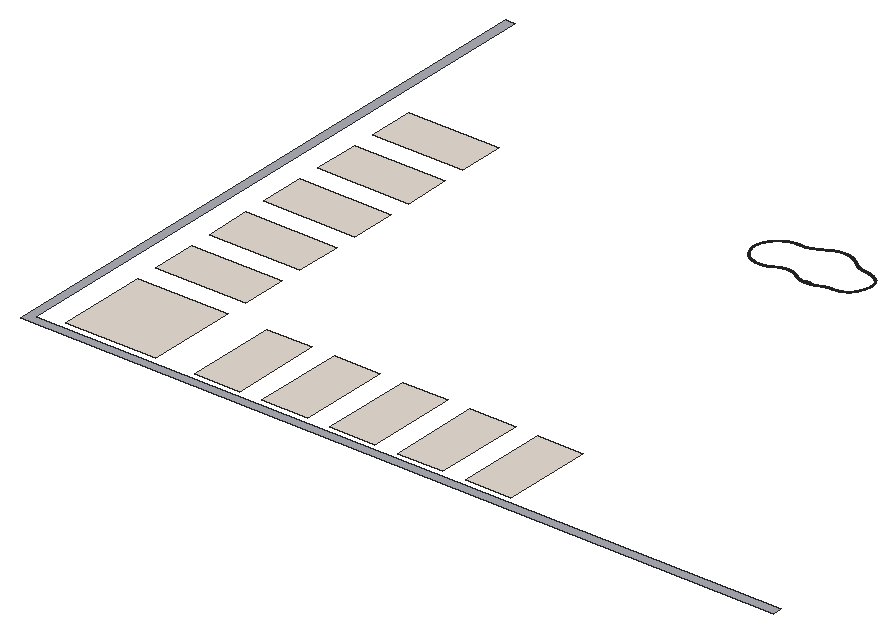
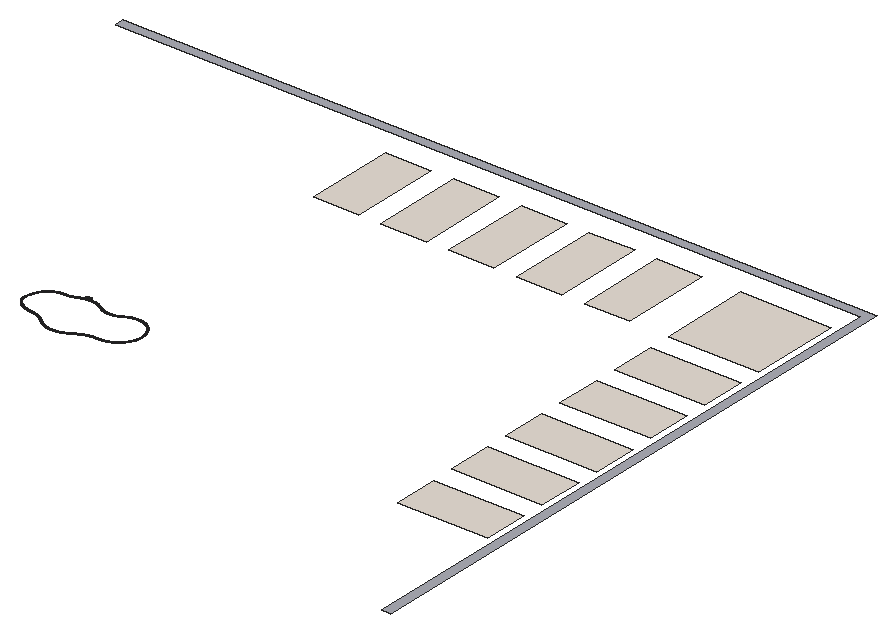
# SketchUp Ruby script. Lengths in inches.
U = 1.inch
M = Sketchup.active_model
def pt(a) = Geom::Point3d.new(a.map { |v| v * U })
def face(e, loops, mat)
  f = e.add_face(loops[0].map { |a| pt(a) })
  loops[1..].each { |l| e.add_face(l.map { |a| pt(a) }).erase! }
  f.material = f.back_material = mat if mat
  f
end
# faces: each face lists its corners as indices into pts; further lists are holes
def faces(e, pts, list, mat = nil) = list.each { |f| face(e, (f[0].is_a?(Array) ? f : [f]).map { |l| l.map { |i| pts[i] } }, mat) }
# xy, xz, yz: faces in a plane at the given z, y or x. An outline is a flat list of corners, or four numbers for a rectangle; further outlines are holes
def ring(l) = l.size == 4 ? [[l[0], l[1]], [l[2], l[1]], [l[2], l[3]], [l[0], l[3]]] : l.each_slice(2).to_a
def flat(e, list, mat, &to3) = list.each { |f| face(e, (f[0].is_a?(Array) ? f : [f]).map { |l| ring(l).map { |u, v| to3.(u, v) } }, mat) }
def xy(e, z, list, mat = nil) = flat(e, list, mat) { |x, y| [x, y, z] }
def xz(e, y, list, mat = nil) = flat(e, list, mat) { |x, z| [x, y, z] }
def yz(e, x, list, mat = nil) = flat(e, list, mat) { |y, z| [x, y, z] }
def lines(e, pts, list) = list.each { |a, b| e.add_line(pt(pts[a]), pt(pts[b])) }
# prism: a flat outline (further loops are holes) pulled along v
def prism(e, loops, v, mat = nil)
  f = face(e, loops, mat); d = Geom::Vector3d.new(v.map { |x| x * U })
  f.pushpull(f.normal.samedirection?(d) ? d.length : -d.length)
end
def box(e, o, s, mat = nil) = prism(e, [[o, [o[0] + s[0], o[1], o[2]], [o[0] + s[0], o[1] + s[1], o[2]], [o[0], o[1] + s[1], o[2]]]], [0, 0, s[2]], mat)
def at(x, y, z, deg = 0) = Geom::Transformation.translation(pt([x, y, z])) * Geom::Transformation.rotation(ORIGIN, Z_AXIS, deg.degrees)
def axes(o, x, y, z) = Geom::Transformation.new([*x, 0, *y, 0, *z, 0, *pt(o).to_a, 1])
def part(name) = M.definitions.add(name)
# library, detail: a bought-in or finely detailed component or shape, given as its bounding box
def library(name, o, s) = part(name).tap { |d| box(d.entities, o, s) }
def detail(e, o, s) = box(e.add_group.entities, o, s)
def put(e, d, t, mat = nil) = e.add_instance(d, t).tap { |i| i.material = mat if mat }
def group(e, t, mat = nil) = e.add_group.tap { |g| g.transformation = t; g.material = mat if mat }.entities
root = M.entities
M.materials.add("Marble_01_1K").color = [230, 221, 211]
M.materials.add("Marble_07_1K").color = [36, 34, 36]
M.materials.add("Marble_20_1K").color = [172, 173, 182]
xy(root,2,[[180.08,576.64,204.08,624.64],[216.08,576.64,240.08,624.64],[252.08,576.64,276.08,624.64],[288.08,576.64,312.08,624.64],[324.08,576.64,348.08,624.64],
  [111.43,576.78,159.43,624.64],[111.43,636.64,159.43,660.64],[111.43,672.64,159.43,696.64],[111.43,708.64,159.43,732.64],[111.43,744.64,159.43,768.64],
  [111.43,780.64,159.43,804.64]],"Marble_01_1K")
xy(root,6,[[98.71,562.78,498.69,562.78,498.69,567.28,103.21,567.28,103.21,885.25,98.71,885.25]],"Marble_20_1K")
xy(root,18,[[[347.23,772.58,347.12,772.59,347,772.59,346.89,772.6,346.78,772.6,346.67,772.61,346.55,772.62,346.22,772.65,346.1,772.67,345.88,772.69,345.55,772.75,345.4375,772.77,345.33,772.79,345.21,772.81,345.1,772.83,344.99,772.86,344.88,772.88,344.77,772.91,344.67,772.93,344.23,773.05,344.12,773.09,344.02,773.12,343.91,773.15,343.69,773.23,343.59,773.26,343.48,773.3,343.27,773.38,343.17,773.43,343.0625,773.47,342.96,773.51,342.86,773.56,342.75,773.6,341.95,774,341.86,774.06,341.76,774.11,341.67,774.16,341.59,774.21,341.51,774.25,341.43,774.3,341.36,774.34,341.24,774.41,341.18,774.45,340.93,774.6,340.89,774.625,340.84,774.65,340.74,774.71,340.7,774.74,340.65,774.76,340.5,774.85,340.4,774.9,340.3,774.96,340.24,774.99,340.18,775.03,340.12,775.06,339.98,775.14,339.89,775.18,339.8,775.23,339.69,775.29,339.17,775.55,339.06,775.6,338.96,775.64,338.8,775.72,338.73,775.75,338.61,775.81,338.55,775.83,338.49,775.86,338.4375,775.88,338.38,775.91,338.18,775.99,338.13,776.02,338.03,776.06,337.97,776.08,337.62,776.22,337.56,776.24,337.21,776.38,337.15,776.4,337.1,776.42,337.06,776.43,336.96,776.47,336.91,776.48,336.86,776.5,336.8,776.52,336.74,776.53,336.66,776.54,336.58,776.56,336.48,776.57,336.36,776.58,336.23,776.6,336.09,776.61,335.9375,776.62,335.78,776.625,335.61,776.63,335.4375,776.64,335.09,776.64,334.91,776.63,334.73,776.63,334.55,776.62,334.2,776.6,334.02,776.58,333.84,776.5625,333.67,776.54,333.49,776.52,333.3125,776.49,333.14,776.46,332.96,776.43,332.79,776.39,332.61,776.36,332.4375,776.32,332.26,776.27,332.09,776.23,331.58,776.08,331.41,776.02,331.24,775.97,331.07,775.91,330.9,775.84,330.74,775.78,330.4,775.64,330.24,775.57,330.08,775.49,329.92,775.42,329.75,775.34,329.59,775.25,329.43,775.17,329.27,775.08,329.1,774.99,328.9375,774.89,328.77,774.8,328.6,774.7,328.42,774.6,328.24,774.49,328.05,774.39,327.87,774.28,327.68,774.18,327.5,774.08,327.32,773.99,327.15,773.9,326.99,773.8125,326.83,773.74,326.68,773.67,326.54,773.61,326.39,773.55,326.23,773.5,325.87,773.4,325.65,773.35,325.42,773.29,325.15,773.24,324.87,773.1875,324.57,773.14,324.26,773.09,323.93,773.05,323.27,772.99,322.93,772.97,322.59,772.96,321.92,772.96,321.58,772.98,321.25,773,320.91,773.04,320.58,773.08,320.24,773.13,319.91,773.1875,319.59,773.25,319.28,773.32,318.97,773.4,318.68,773.47,318.41,773.55,318.16,773.63,317.92,773.71,317.71,773.79,317.51,773.87,317.32,773.96,317.13,774.04,316.96,774.14,316.78,774.24,316.61,774.34,316.43,774.46,316.24,774.59,316.03,774.74,315.81,774.9,315.57,775.1,315.3,775.33,314.99,775.59,314.66,775.89,314.36,776.24,314.11,776.54,313.89,776.82,313.7,777.0625,313.54,777.28,313.4,777.48,313.27,777.67,313.16,777.84,313.06,778.01,312.96,778.17,312.78,778.47,312.7,778.62,312.63,778.77,312.49,779.05,312.35,779.35,312.29,779.49,312.05,780.09,311.95,780.39,311.9,780.55,311.85,780.7,311.81,780.85,311.76,781.01,311.72,781.16,311.68,781.32,311.65,781.47,311.61,781.63,311.58,781.79,311.55,781.9375,311.52,782.09,311.48,782.37,311.46,782.5,311.4375,782.625,311.42,782.74,311.41,782.84,311.4,782.9375,311.39,783.03,311.39,783.12,311.38,783.2,311.38,783.28,311.37,783.36,311.37,783.45,311.36,783.53,311.36,783.71,311.35,783.81,311.35,784.27,311.36,784.4,311.36,784.54,311.37,784.6875,311.38,784.84,311.39,784.99,311.41,785.15,311.42,785.3,311.48,785.78,311.51,785.9375,311.54,786.09,311.56,786.25,311.6,786.41,311.63,786.57,311.75,787.05,311.8,787.22,311.86,787.39,311.92,787.57,311.99,787.75,312.07,787.94,312.16,788.14,312.26,788.35,312.48,788.77,312.72,789.19,312.83,789.39,312.95,789.59,313.0625,789.78,313.17,789.96,313.28,790.13,313.39,790.29,313.49,790.45,313.6,790.6,313.7,790.75,313.8125,790.9,313.92,791.05,314.03,791.19,314.15,791.34,314.26,791.48,314.74,792.04,314.87,792.17,314.99,792.3,315.12,792.43,315.25,792.5625,315.38,792.69,315.51,792.82,315.65,792.94,315.79,793.0625,315.92,793.19,316.0625,793.3,316.2,793.42,316.35,793.54,316.49,793.65,316.64,793.76,316.78,793.87,316.93,793.98,317.08,794.08,317.23,794.1875,317.39,794.29,317.54,794.39,317.7,794.48,317.85,794.58,318.65,795.03,318.82,795.11,318.98,795.1875,319.15,795.27,319.32,795.34,319.48,795.42,319.82,795.56,320.16,795.69,320.34,795.75,320.51,795.8125,320.68,795.87,320.86,795.93,321.03,795.98,321.39,796.08,321.5625,796.125,321.74,796.17,322.28,796.29,322.46,796.32,322.64,796.36,322.82,796.39,323,796.41,323.18,796.4375,323.37,796.46,323.73,796.5,323.92,796.51,324.1,796.53,324.28,796.54,324.45,796.55,324.62,796.55,324.78,796.56,325.33,796.56,325.4375,796.55,325.54,796.55,325.64,796.54,325.73,796.53,325.82,796.53,325.9,796.52,325.99,796.52,326.07,796.51,326.16,796.51,326.25,796.5,326.52,796.5,326.62,796.49,326.97,796.49,327.11,796.5,327.27,796.5,327.45,796.51,327.65,796.52,327.88,796.53,328.11,796.56,328.3125,796.58,328.49,796.6,328.65,796.625,328.79,796.65,328.91,796.67,329.02,796.68,329.13,796.7,329.23,796.72,329.41,796.76,329.5,796.77,329.98,796.89,330.0625,796.91,330.14,796.93,330.46,797.01,330.54,797.04,330.62,797.06,330.69,797.08,330.77,797.11,330.85,797.13,330.93,797.16,331.01,797.1875,331.08,797.21,331.24,797.27,331.32,797.29,331.39,797.32,331.55,797.38,331.62,797.41,331.78,797.47,331.85,797.5,331.93,797.54,332,797.57,332.08,797.6,332.15,797.63,332.23,797.67,332.31,797.7,332.38,797.74,332.46,797.77,332.54,797.8125,332.625,797.85,332.71,797.9,332.81,797.94,332.91,797.99,333.02,798.04,333.14,798.1,333.27,798.16,333.41,798.22,333.55,798.29,333.85,798.43,334.01,798.5,334.16,798.57,334.31,798.65,334.47,798.72,334.62,798.8,334.77,798.87,334.92,798.95,335.08,799.02,335.23,799.1,335.375,799.18,335.53,799.26,335.83,799.42,335.97,799.5,336.27,799.66,336.42,799.75,336.57,799.83,336.71,799.91,336.86,800,337,800.08,337.13,800.16,337.26,800.23,337.375,800.3,337.48,800.37,337.57,800.42,337.65,800.47,337.72,800.51,337.78,800.54,337.86,800.6,337.89,800.62,337.93,800.64,337.95,800.66,338.01,800.7,338.04,800.71,338.07,800.73,338.11,800.75,338.14,800.77,338.17,800.8,338.25,800.84,338.29,800.87,338.34,800.89,338.39,800.92,338.45,800.96,338.59,801.04,338.68,801.09,338.77,801.13,338.85,801.17,338.92,801.21,338.98,801.24,339.03,801.27,339.08,801.29,339.125,801.3125,339.17,801.33,339.21,801.35,339.24,801.37,339.28,801.39,339.3125,801.4,339.35,801.42,339.38,801.43,339.41,801.45,339.44,801.46,339.48,801.48,339.54,801.5,339.57,801.52,339.61,801.53,339.64,801.54,339.67,801.56,339.71,801.57,339.74,801.59,339.8,801.61,339.84,801.625,339.87,801.64,339.9,801.65,339.94,801.66,339.97,801.68,340.03,801.7,340.07,801.71,340.1,801.73,340.13,801.74,340.17,801.75,340.23,801.77,340.27,801.79,340.33,801.81,340.37,801.82,340.4,801.83,340.44,801.84,340.47,801.86,340.5,801.87,340.54,801.88,340.57,801.89,340.61,801.9,340.66,801.92,340.72,801.93,340.79,801.95,340.87,801.97,340.96,802,341.07,802.03,341.21,802.07,341.36,802.11,341.55,802.15,341.76,802.2,342.01,802.26,342.3,802.32,342.63,802.39,342.99,802.4375,343.34,802.47,343.67,802.5,343.99,802.51,344.29,802.52,344.58,802.52,344.85,802.51,345.11,802.5,345.34,802.49,345.56,802.48,345.76,802.47,345.9375,802.46,346.1,802.45,346.25,802.4375,346.38,802.43,346.49,802.42,346.59,802.41,346.67,802.4,346.74,802.39,346.8,802.39,346.85,802.38,346.89,802.38,346.97,802.37,347.01,802.36,347.05,802.36,347.09,802.35,347.125,802.35,347.16,802.34,347.2,802.34,347.24,802.33,347.28,802.33,347.35,802.3125,347.39,802.31,347.43,802.3,347.47,802.3,347.55,802.28,347.58,802.27,347.62,802.27,347.74,802.24,347.78,802.24,347.8125,802.23,347.85,802.22,347.97,802.19,348,802.19,348.08,802.17,348.125,802.16,348.17,802.14,348.22,802.13,348.26,802.12,348.32,802.11,348.375,802.09,348.4375,802.07,348.51,802.05,348.59,802.03,348.68,802,348.79,801.97,348.89,801.93,348.98,801.9,349.0625,801.87,349.13,801.84,349.2,801.82,349.35,801.76,349.43,801.72,349.47,801.71,349.51,801.69,349.55,801.68,349.59,801.66,349.62,801.64,349.66,801.63,349.69,801.61,349.73,801.6,349.76,801.58,349.8,801.56,349.83,801.55,349.91,801.51,349.94,801.5,349.97,801.48,350.01,801.46,350.05,801.45,350.08,801.43,350.16,801.39,350.21,801.36,350.25,801.34,350.3,801.3125,350.35,801.29,350.41,801.26,350.46,801.23,350.52,801.2,350.58,801.16,350.7,801.1,350.76,801.06,350.82,801.03,350.875,801,350.93,800.96,351.05,800.9,351.11,800.86,351.17,800.83,351.23,800.79,351.29,800.76,351.34,800.72,351.4,800.6875,351.46,800.65,351.52,800.62,351.58,800.58,351.63,800.54,351.69,800.51,351.75,800.47,351.81,800.4375,351.86,800.4,351.92,800.36,351.98,800.33,352.04,800.29,352.09,800.25,352.15,800.21,352.21,800.18,352.26,800.14,352.32,800.1,352.38,800.05,352.45,800.01,352.51,799.97,352.65,799.87,352.73,799.8125,352.81,799.75,352.91,799.6875,353.02,799.61,353.14,799.52,353.27,799.42,353.42,799.3,353.57,799.19,353.71,799.08,353.93,798.9,354.02,798.82,354.29,798.61,354.46,798.47,354.55,798.4,354.65,798.33,354.74,798.25,354.84,798.18,354.9375,798.11,355.04,798.04,355.13,797.97,355.43,797.76,355.53,797.7,355.64,797.63,355.84,797.51,355.94,797.44,356.05,797.38,356.15,797.32,356.26,797.27,356.36,797.21,356.47,797.15,356.58,797.1,356.68,797.04,356.79,796.99,356.9,796.9375,357.01,796.89,357.45,796.69,357.5625,796.65,357.68,796.6,357.79,796.5625,357.9,796.52,358.01,796.48,358.13,796.4375,358.24,796.4,358.36,796.36,358.47,796.33,358.59,796.29,358.7,796.26,358.82,796.23,358.93,796.19,359.05,796.16,359.17,796.14,359.28,796.11,359.4,796.08,359.52,796.06,359.64,796.03,359.76,796.01,359.99,795.97,360.47,795.89,360.71,795.87,360.83,795.85,360.95,795.84,361.17,795.82,361.47,795.79,361.56,795.78,361.65,795.78,361.81,795.76,361.9,795.75,361.98,795.74,362.0625,795.73,362.15,795.73,362.23,795.71,362.3125,795.7,362.39,795.69,362.48,795.68,362.64,795.66,362.73,795.64,362.81,795.63,362.89,795.61,362.97,795.6,363.06,795.58,363.14,795.57,363.3,795.53,363.39,795.52,363.63,795.46,363.71,795.4375,363.8,795.42,363.88,795.4,364.04,795.35,364.28,795.29,364.36,795.26,364.44,795.24,364.52,795.21,364.6,795.1875,364.68,795.16,364.76,795.13,364.84,795.11,365.4,794.9,365.48,794.875,365.55,794.84,365.71,794.78,365.79,794.74,365.86,794.71,365.94,794.68,366.02,794.64,366.09,794.61,366.17,794.57,366.25,794.54,366.32,794.5,366.4,794.46,366.47,794.43,366.55,794.39,366.62,794.35,366.7,794.31,366.77,794.27,366.85,794.23,366.99,794.15,367.07,794.11,367.21,794.03,367.28,793.98,367.36,793.9375,367.43,793.9,367.5,793.85,367.57,793.81,367.64,793.76,367.71,793.72,367.78,793.67,367.92,793.59,367.98,793.55,368.08,793.47,368.125,793.44,368.16,793.42,368.22,793.38,368.24,793.37,368.25,793.35,368.27,793.34,368.28,793.34,368.3,793.32,368.32,793.31,368.33,793.3,368.35,793.29,368.38,793.26,368.41,793.24,368.43,793.22,368.46,793.2,368.5,793.18,368.53,793.15,368.61,793.09,368.66,793.05,368.7,793.02,368.8,792.94,368.84,792.91,368.89,792.87,368.9375,792.83,368.99,792.79,369.03,792.75,369.13,792.67,369.23,792.58,369.32,792.49,369.37,792.45,369.41,792.4,369.46,792.36,369.51,792.3125,369.55,792.26,369.64,792.17,369.68,792.12,369.73,792.07,370.05,791.67,370.09,791.61,370.125,791.5625,370.16,791.51,370.2,791.46,370.24,791.4,370.27,791.35,370.31,791.29,370.34,791.24,370.375,791.18,370.41,791.125,370.44,791.07,370.47,791.01,370.51,790.96,370.625,790.73,370.65,790.67,370.74,790.49,370.76,790.43,370.79,790.375,370.8125,790.3125,370.84,790.25,370.86,790.19,370.89,790.13,370.99,789.83,371.01,789.76,371.07,789.58,371.08,789.51,371.12,789.39,371.13,789.32,371.14,789.26,371.16,789.2,371.17,789.13,371.18,789.07,371.2,789.01,371.21,788.94,371.22,788.88,371.23,788.81,371.24,788.75,371.24,788.6875,371.25,788.62,371.26,788.56,371.27,788.49,371.27,788.43,371.28,788.36,371.28,788.23,371.29,788.17,371.29,787.78,371.28,787.65,371.26,787.49,371.25,787.3,371.22,787.07,371.19,786.79,371.15,786.45,371.09,786.06,371.01,785.59,370.9,785.05,370.76,784.42,370.59,783.7,370.37,782.88,370.02,782.11,369.7,781.4375,369.4,780.85,369.11,780.34,368.85,779.9,368.59,779.52,368.35,779.18,368.11,778.875,367.875,778.6,367.64,778.35,367.41,778.11,367.17,777.9,366.9375,777.7,366.7,777.52,366.22,777.18,365.98,777.02,365.48,776.73,365.22,776.59,364.96,776.46,364.7,776.34,364.4375,776.22,364.17,776.11,363.9,776.01,363.625,775.91,363.35,775.82,363.08,775.74,362.8,775.66,362.52,775.59,362.24,775.53,361.96,775.48,361.67,775.43,361.39,775.39,360.85,775.33,360.6,775.31,360.36,775.29,360.14,775.27,359.9375,775.26,359.76,775.25,359.6,775.25,359.46,775.24,359.22,775.24,359.12,775.23,358.84,775.23,358.74,775.22,358.65,775.22,358.5625,775.21,358.47,775.21,358.38,775.2,358.29,775.2,358.2,775.1875,358.11,775.18,357.48,775.11,357.39,775.09,357.3,775.08,357.22,775.07,357.125,775.05,357.04,775.04,356.77,774.98,356.68,774.97,356.6,774.95,356.24,774.87,356.16,774.85,356.07,774.82,355.89,774.78,355.81,774.75,355.72,774.73,355.63,774.7,355.55,774.68,355.46,774.65,355.29,774.59,355.2,774.5625,355.12,774.54,355.03,774.51,354.95,774.47,354.86,774.44,354.78,774.41,354.69,774.38,354.61,774.35,354.52,774.3125,354.4375,774.28,354.35,774.24,354.19,774.18,354.11,774.14,353.95,774.08,353.875,774.04,353.8,774.01,353.73,773.98,353.65,773.95,353.51,773.89,353.4375,773.86,353.36,773.83,353.22,773.77,353.14,773.74,353.07,773.71,352.99,773.68,352.92,773.65,352.84,773.625,352.77,773.6,352.69,773.57,352.62,773.54,352.54,773.52,352.47,773.49,352.39,773.47,352.32,773.44,352.24,773.42,352.17,773.39,352.09,773.37,352.01,773.34,351.9375,773.32,351.86,773.29,351.79,773.27,351.63,773.23,351.56,773.2,351.4,773.16,351.33,773.14,351.09,773.08,351.02,773.06,350.9375,773.04,350.86,773.02,350.78,773,350.71,772.98,350.63,772.96,350.55,772.95,350.47,772.93,350.4,772.91,350.32,772.9,350.16,772.86,350.08,772.85,350,772.83,349.93,772.82,349.85,772.8,349.77,772.79,349.6875,772.78,349.61,772.76,349.45,772.74,349.36,772.72,349.28,772.71,349.18,772.7,349.09,772.69,348.99,772.67,348.79,772.65,348.24,772.6,348.13,772.6,348.02,772.59,347.79,772.58],[347.35,773.18,347.67,773.18,347.88,773.19,347.99,773.19,348.1,773.2,348.2,773.21,348.31,773.21,348.42,773.22,348.52,773.23,348.73,773.25,348.83,773.26,349.01,773.28,349.1,773.3,349.19,773.31,349.43,773.34,349.51,773.36,349.59,773.37,349.66,773.38,349.74,773.4,349.81,773.41,349.89,773.43,349.97,773.44,350.04,773.46,350.12,773.47,350.19,773.49,350.27,773.5,350.34,773.52,350.42,773.54,350.49,773.55,350.57,773.57,350.64,773.59,350.72,773.61,350.79,773.625,350.87,773.64,350.94,773.66,351.02,773.68,351.09,773.7,351.17,773.72,351.24,773.74,351.32,773.76,351.39,773.78,351.46,773.81,351.54,773.83,351.68,773.87,351.76,773.89,351.83,773.92,351.91,773.94,351.98,773.96,352.05,773.99,352.125,774.01,352.2,774.04,352.27,774.0625,352.34,774.09,352.42,774.11,352.49,774.14,352.5625,774.17,352.63,774.19,352.71,774.22,352.78,774.25,352.85,774.27,352.99,774.33,353.07,774.36,353.42,774.51,353.5,774.54,353.64,774.6,353.72,774.63,353.8,774.67,353.96,774.73,354.04,774.77,354.13,774.8,354.21,774.84,354.39,774.91,354.48,774.94,354.57,774.98,354.65,775.01,354.83,775.07,354.92,775.11,355.19,775.2,355.28,775.22,355.55,775.31,355.64,775.33,355.73,775.36,355.82,775.38,355.92,775.41,356.1,775.45,356.19,775.48,356.28,775.5,356.47,775.54,356.65,775.58,356.75,775.59,356.84,775.61,356.94,775.63,357.03,775.65,357.13,775.66,357.35,775.7,357.46,775.71,357.58,775.73,357.71,775.74,357.86,775.76,358.02,775.78,358.2,775.79,358.4,775.81,358.64,775.82,358.9,775.84,359.2,775.84,359.53,775.85,359.87,775.87,360.59,775.93,360.96,775.97,361.31,776.01,361.66,776.06,361.99,776.11,362.3,776.18,362.6,776.24,362.89,776.32,363.16,776.39,363.43,776.48,363.69,776.57,363.95,776.67,364.2,776.77,364.45,776.89,364.7,777,364.94,777.125,365.18,777.26,365.42,777.39,365.65,777.53,366.11,777.83,366.33,777.99,366.55,778.16,366.76,778.33,366.97,778.51,367.17,778.7,367.55,779.1,367.91,779.54,368.23,780,368.39,780.24,368.53,780.49,368.68,780.74,368.82,780.99,369.08,781.51,369.32,782.03,369.43,782.3,369.54,782.5625,369.65,782.83,369.75,783.1,369.93,783.65,370.01,783.93,370.09,784.2,370.17,784.48,370.23,784.76,370.3,785.04,370.36,785.33,370.46,785.89,370.54,786.43,370.57,786.68,370.6,786.91,370.625,787.12,370.64,787.31,370.66,787.47,370.67,787.6,370.68,787.72,370.69,787.8125,370.6875,787.89,370.6875,788.08,370.68,788.14,370.68,788.26,370.67,788.32,370.67,788.38,370.66,788.4375,370.66,788.49,370.65,788.55,370.65,788.61,370.62,788.79,370.61,788.84,370.58,789.02,370.57,789.07,370.56,789.13,370.54,789.1875,370.53,789.25,370.51,789.3,370.5,789.36,370.48,789.42,370.47,789.47,370.45,789.53,370.44,789.59,370.42,789.64,370.4,789.7,370.38,789.75,370.36,789.81,370.34,789.86,370.32,789.92,370.3,789.97,370.28,790.03,370.26,790.08,370.23,790.14,370.21,790.19,370.1875,790.25,370.16,790.3,370.14,790.35,370.11,790.41,370.09,790.46,370.06,790.51,370.03,790.5625,370.01,790.61,369.98,790.67,369.77,791.02,369.73,791.07,369.67,791.17,369.63,791.21,369.57,791.31,369.53,791.36,369.49,791.4,369.46,791.45,369.42,791.49,369.38,791.54,369.35,791.59,369.27,791.67,369.23,791.72,369.19,791.76,369.15,791.81,368.99,791.97,368.95,792.02,368.91,792.06,368.86,792.1,368.78,792.18,368.73,792.21,368.6875,792.25,368.64,792.29,368.6,792.33,368.55,792.37,368.46,792.4375,368.42,792.47,368.375,792.51,368.33,792.54,368.29,792.58,368.17,792.67,368.13,792.69,368.1,792.72,368.07,792.74,368.05,792.76,368.03,792.77,368.01,792.79,367.99,792.8,367.98,792.8125,367.96,792.82,367.95,792.83,367.9375,792.84,367.93,792.85,367.92,792.86,367.9,792.86,367.89,792.875,367.87,792.89,367.78,792.95,367.74,792.98,367.69,793.01,367.64,793.05,367.58,793.08,367.52,793.125,367.45,793.17,367.39,793.21,367.32,793.25,367.25,793.3,367.11,793.38,367.05,793.42,366.42,793.78,366.35,793.8125,366.27,793.85,366.2,793.89,366.13,793.92,366.06,793.96,365.99,793.99,365.91,794.03,365.77,794.09,365.69,794.125,365.62,794.16,365.55,794.19,365.47,794.22,365.33,794.28,365.25,794.3125,365.18,794.34,365.1,794.37,365.03,794.4,364.95,794.43,364.875,794.46,364.8,794.48,364.72,794.51,364.65,794.54,364.57,794.5625,364.5,794.59,364.42,794.61,364.34,794.64,364.27,794.66,364.19,794.68,364.11,794.71,364.04,794.73,363.8,794.79,363.73,794.8125,363.65,794.83,363.41,794.89,363.34,794.91,363.26,794.93,363.18,794.94,363.1,794.96,363.02,794.97,362.94,794.99,362.86,795,362.79,795.02,362.71,795.03,362.63,795.05,362.39,795.08,362.31,795.1,362.15,795.12,362.07,795.125,361.99,795.14,361.91,795.14,361.67,795.17,361.58,795.18,361.5,795.18,361.41,795.19,361.3125,795.2,361.21,795.21,361.11,795.22,360.99,795.23,360.88,795.24,360.76,795.25,360.64,795.27,360.52,795.28,360.39,795.3,360.27,795.3125,360.14,795.33,360.02,795.35,359.89,795.37,359.77,795.39,359.64,795.42,359.52,795.44,359.39,795.47,359.27,795.49,359.15,795.52,359.02,795.55,358.66,795.64,358.54,795.68,358.41,795.71,357.93,795.87,357.8125,795.91,357.69,795.95,357.58,796,357.46,796.04,357.22,796.14,357.11,796.18,356.99,796.23,356.875,796.29,356.76,796.34,356.64,796.39,356.53,796.45,356.42,796.5,356.3,796.56,355.64,796.92,355.53,796.99,355.42,797.05,355.3125,797.12,355.21,797.19,355.1,797.26,355,797.33,354.89,797.4,354.79,797.47,354.69,797.55,354.58,797.62,354.48,797.69,354.38,797.77,354.02,798.05,353.94,798.11,353.87,798.17,353.81,798.22,353.74,798.27,353.68,798.32,353.63,798.37,353.57,798.41,353.52,798.45,353.47,798.5,353.32,798.62,353.26,798.66,353.06,798.82,353,798.86,352.9,798.94,352.84,798.98,352.79,799.02,352.74,799.0625,352.68,799.1,352.58,799.18,352.52,799.22,352.42,799.3,352.36,799.34,352.31,799.375,352.25,799.41,352.15,799.49,352.09,799.52,352.04,799.5625,351.98,799.6,351.93,799.64,351.87,799.67,351.82,799.71,351.76,799.75,351.71,799.78,351.65,799.82,351.59,799.85,351.54,799.89,351.48,799.93,351.43,799.96,351.37,800,351.31,800.03,351.26,800.07,351.2,800.1,351.15,800.14,351.09,800.17,351.03,800.21,350.98,800.24,350.92,800.27,350.86,800.31,350.8,800.34,350.75,800.375,350.69,800.41,350.63,800.44,350.58,800.47,350.52,800.51,350.34,800.6,350.29,800.63,350.23,800.67,350.17,800.7,350.12,800.73,350.07,800.75,350.02,800.78,349.97,800.8,349.93,800.83,349.85,800.87,349.8125,800.89,349.78,800.91,349.74,800.92,349.71,800.9375,349.68,800.95,349.64,800.97,349.61,800.99,349.58,801,349.55,801.02,349.51,801.03,349.48,801.05,349.45,801.0625,349.41,801.08,349.38,801.09,349.35,801.11,349.3125,801.12,349.28,801.14,349.25,801.15,349.21,801.16,349.18,801.18,349.15,801.19,349.11,801.2,349.08,801.22,349.04,801.23,349.01,801.24,348.98,801.26,348.94,801.27,348.91,801.28,348.875,801.3,348.84,801.31,348.81,801.32,348.77,801.33,348.74,801.34,348.7,801.36,348.67,801.37,348.63,801.38,348.6,801.39,348.56,801.4,348.5,801.42,348.46,801.44,348.43,801.45,348.39,801.46,348.36,801.47,348.32,801.48,348.29,801.49,348.25,801.5,348.22,801.51,348.18,801.52,348.15,801.53,348.11,801.54,348.08,801.55,348.04,801.55,348.01,801.5625,347.97,801.57,347.94,801.58,347.86,801.6,347.83,801.61,347.79,801.61,347.76,801.62,347.72,801.63,347.6875,801.64,347.65,801.65,347.62,801.65,347.54,801.67,347.51,801.67,347.47,801.68,347.4375,801.6875,347.4,801.69,347.37,801.7,347.33,801.71,347.29,801.71,347.26,801.72,347.22,801.72,347.1875,801.73,347.15,801.74,347.11,801.74,347.08,801.75,347.04,801.75,347.01,801.76,346.97,801.76,346.93,801.77,346.86,801.77,346.2,801.84,346.0625,801.85,345.91,801.86,345.59,801.88,345.23,801.9,345.04,801.91,344.85,801.91,344.66,801.92,344.1,801.92,343.93,801.91,343.77,801.91,343.61,801.9,343.47,801.89,343.21,801.86,343.09,801.84,342.97,801.83,342.85,801.81,342.74,801.79,342.51,801.75,342.4,801.72,342.29,801.7,342.17,801.68,342.0625,801.65,341.95,801.63,341.84,801.6,341.72,801.57,341.61,801.55,341.51,801.52,341.4,801.49,341.3,801.47,341.21,801.44,341.125,801.42,341.05,801.4,340.98,801.38,340.92,801.36,340.83,801.34,340.79,801.32,340.75,801.3125,340.72,801.3,340.6875,801.29,340.66,801.28,340.59,801.26,340.5625,801.25,340.53,801.24,340.44,801.21,340.4,801.19,340.25,801.14,340.22,801.125,340.18,801.11,340.09,801.08,340.06,801.0625,340.02,801.05,339.99,801.04,339.95,801.02,339.92,801.01,339.83,800.97,339.79,800.95,339.73,800.93,339.61,800.87,339.53,800.84,339.45,800.8,339.36,800.76,339.29,800.72,339.22,800.6875,339.16,800.66,339.11,800.63,338.95,800.55,338.89,800.51,338.85,800.49,338.82,800.48,338.76,800.44,338.73,800.43,338.71,800.41,338.68,800.39,338.62,800.36,338.59,800.34,338.5625,800.32,338.53,800.31,338.5,800.29,338.48,800.27,338.45,800.25,338.42,800.24,338.33,800.18,338.31,800.17,338.22,800.11,338.18,800.09,338.14,800.0625,338.1,800.03,338.04,800,337.97,799.96,337.89,799.91,337.8,799.85,337.6875,799.79,337.57,799.72,337.44,799.64,337.16,799.48,336.86,799.3,336.71,799.22,336.5625,799.13,336.41,799.05,336.25,798.96,336.09,798.875,335.92,798.78,335.74,798.69,335.36,798.49,335.14,798.38,334.91,798.27,334.64,798.14,334.34,797.99,334,797.83,333.61,797.65,333.17,797.45,332.96,797.34,332.76,797.25,332.59,797.17,332.44,797.1,332.31,797.04,332.1875,796.99,332.08,796.95,331.98,796.9,331.88,796.87,331.7,796.79,331.61,796.76,331.53,796.73,331.44,796.7,331.2,796.61,331.12,796.59,331.04,796.56,330.95,796.53,330.875,796.51,330.79,796.48,330.71,796.46,330.625,796.43,330.54,796.41,330.46,796.39,330.38,796.36,330.3,796.34,330.21,796.32,330.05,796.28,329.96,796.26,329.8,796.22,329.71,796.2,329.63,796.18,329.54,796.17,329.46,796.15,329.375,796.13,329.29,796.12,329.21,796.1,329.12,796.09,329.04,796.07,328.95,796.06,328.87,796.05,328.78,796.03,328.7,796.02,328.61,796.01,328.53,796,328.44,795.99,328.36,795.98,328.27,795.97,328.1875,795.96,328.1,795.95,328.02,795.94,327.93,795.9375,327.84,795.93,327.76,795.92,327.67,795.92,327.59,795.91,327.5,795.91,327.42,795.9,327.24,795.9,327.16,795.89,326.39,795.89,326.3,795.9,326.13,795.9,326.04,795.91,325.96,795.91,325.87,795.92,325.79,795.92,325.7,795.93,325.61,795.9375,325.52,795.94,325.42,795.95,325.19,795.95,325.07,795.96,324.93,795.96,324.79,795.95,324.63,795.95,324.47,795.94,324.3,795.94,324.13,795.92,323.79,795.9,323.61,795.88,323.4375,795.86,323.26,795.84,323.09,795.82,322.92,795.79,322.74,795.76,322.4,795.7,322.23,795.66,322.05,795.625,321.88,795.58,321.54,795.5,321.21,795.4,320.87,795.3,320.7,795.24,320.54,795.18,320.375,795.125,320.21,795.0625,320.05,795,319.88,794.93,319.72,794.86,319.5625,794.79,319.4,794.72,319.24,794.64,319.09,794.57,318.77,794.41,318.62,794.32,318.47,794.24,318.3125,794.15,318.16,794.0625,318.01,793.97,317.86,793.88,317.72,793.78,317.57,793.6875,317.43,793.59,317.28,793.49,317.14,793.38,317,793.28,316.86,793.17,316.72,793.0625,316.59,792.95,316.45,792.84,316.32,792.73,316.19,792.61,316.05,792.5,315.93,792.375,315.8,792.26,315.55,792.01,315.43,791.88,315.31,791.76,315.1875,791.63,315.07,791.5,314.95,791.37,314.84,791.23,314.73,791.1,314.4,790.68,314.3,790.54,314.19,790.4,314.09,790.26,313.89,789.96,313.79,789.8,313.68,789.64,313.58,789.46,313.36,789.1,313.25,788.9,313.13,788.7,313.02,788.5,312.92,788.3,312.8125,788.1,312.72,787.9,312.63,787.71,312.55,787.53,312.49,787.36,312.43,787.2,312.375,787.04,312.33,786.88,312.25,786.58,312.22,786.43,312.1875,786.29,312.16,786.14,312.1,785.84,312.08,785.6875,312.06,785.54,312.04,785.39,312.02,785.23,312.01,785.08,311.99,784.93,311.97,784.63,311.97,784.48,311.96,784.32,311.96,783.87,311.97,783.72,311.97,783.5625,311.98,783.41,312,783.11,312.02,782.96,312.03,782.81,312.07,782.51,312.09,782.35,312.12,782.2,312.14,782.05,312.17,781.91,312.2,781.76,312.24,781.61,312.27,781.46,312.31,781.3125,312.35,781.16,312.39,781.01,312.4375,780.85,312.49,780.6875,312.55,780.52,312.61,780.35,312.68,780.16,312.75,779.96,312.84,779.75,312.95,779.51,313.07,779.25,313.39,778.61,313.59,778.23,313.84,777.88,314.0625,777.58,314.26,777.3125,314.45,777.08,314.61,776.88,314.76,776.71,314.91,776.55,315.04,776.41,315.17,776.28,315.29,776.15,315.42,776.03,315.54,775.92,315.65,775.8125,315.77,775.71,315.89,775.61,316,775.51,316.12,775.41,316.36,775.23,316.49,775.14,316.61,775.05,316.74,774.96,317,774.8,317.28,774.64,317.43,774.57,317.59,774.49,317.76,774.42,317.94,774.35,318.14,774.27,318.36,774.2,318.6,774.125,318.86,774.05,319.13,773.98,319.42,773.91,319.72,773.84,320.34,773.72,321.3,773.6,321.62,773.58,322.26,773.56,322.58,773.56,322.91,773.57,323.23,773.59,323.55,773.62,323.86,773.65,324.17,773.6875,324.47,773.73,324.76,773.78,325.02,773.83,325.27,773.88,325.5,773.93,325.69,773.98,325.87,774.02,326.03,774.07,326.18,774.12,326.32,774.17,326.45,774.23,326.59,774.29,326.74,774.36,326.89,774.44,327.23,774.62,327.77,774.92,327.95,775.03,328.31,775.23,328.65,775.43,328.99,775.61,329.15,775.7,329.49,775.88,329.65,775.96,329.99,776.12,330.17,776.2,330.51,776.34,330.6875,776.41,330.86,776.47,331.04,776.54,331.22,776.6,331.39,776.65,331.57,776.71,331.75,776.76,331.93,776.8125,332.12,776.86,332.3,776.9,332.48,776.95,332.66,776.98,332.85,777.02,333.03,777.05,333.22,777.08,333.4,777.11,333.59,777.14,333.78,777.16,333.96,777.18,334.15,777.2,334.34,777.21,334.52,777.22,334.9,777.24,335.46,777.24,335.64,777.23,335.82,777.23,336,777.22,336.17,777.21,336.32,777.19,336.46,777.18,336.59,777.17,336.71,777.15,336.8,777.13,336.89,777.12,337.03,777.08,337.09,777.0625,337.15,777.04,337.2,777.02,337.25,777.01,337.31,776.99,337.41,776.95,337.47,776.93,337.57,776.89,337.68,776.85,337.78,776.81,337.84,776.79,337.89,776.76,337.99,776.72,338.05,776.7,338.2,776.64,338.26,776.62,338.31,776.59,338.41,776.55,338.47,776.53,338.52,776.51,338.57,776.48,338.62,776.46,338.67,776.4375,338.73,776.42,338.78,776.39,338.88,776.35,338.93,776.32,338.98,776.3,339.04,776.28,339.09,776.25,339.14,776.23,339.19,776.2,339.29,776.16,339.34,776.13,339.4,776.11,339.45,776.08,339.5,776.06,339.55,776.03,339.6,776.01,339.65,775.98,339.7,775.96,339.75,775.93,339.8,775.91,339.85,775.88,339.9,775.86,340,775.8,340.05,775.78,340.1,775.75,340.16,775.73,340.26,775.67,340.31,775.65,340.41,775.59,340.45,775.57,340.6,775.48,340.65,775.46,340.85,775.34,340.9,775.32,341.15,775.17,341.19,775.14,341.24,775.12,341.44,775,341.49,774.96,341.61,774.9,341.67,774.86,341.74,774.82,341.8125,774.78,341.89,774.73,341.97,774.68,342.33,774.48,342.43,774.43,342.52,774.38,342.62,774.34,342.71,774.29,342.81,774.24,342.9,774.2,343,774.15,343.3,774.03,343.39,773.99,343.79,773.83,343.89,773.8,343.99,773.76,344.1,773.73,344.2,773.7,344.3,773.66,344.5,773.6,344.61,773.57,344.71,773.55,344.8125,773.52,344.92,773.49,345.02,773.47,345.125,773.45,345.23,773.42,345.33,773.4,345.4375,773.38,345.54,773.36,345.65,773.34,345.75,773.32,345.86,773.31,345.97,773.29,346.07,773.28,346.18,773.26,346.28,773.25,346.5,773.23,346.6,773.22,346.71,773.21,346.82,773.21,346.92,773.2,347.03,773.19,347.14,773.19,347.24,773.1875]]],"Marble_07_1K")
xz(root,772.58,[[347.34,18,347.57,19],[347.57,18,347.68,19],[347.68,18,347.79,19]],"Marble_07_1K")
xz(root,772.6,[[348.13,18,348.24,19]],"Marble_07_1K")
p = [[347.79,772.58,18],[348.02,772.59,18],[348.02,772.59,19],[347.79,772.58,19],[348.13,772.6,18],[348.13,772.6,19],
  [348.24,772.6,18],[348.35,772.61,18],[348.35,772.61,19],[348.24,772.6,19],[348.46,772.62,18],[348.46,772.62,19],
  [348.57,772.63,18],[348.57,772.63,19],[348.68,772.64,18],[348.68,772.64,19],[348.79,772.65,18],[348.79,772.65,19],
  [348.89,772.66,18],[348.89,772.66,19],[348.99,772.67,18],[348.99,772.67,19],[349.09,772.69,18],[349.09,772.69,19],
  [349.18,772.7,18],[349.18,772.7,19],[349.28,772.71,18],[349.28,772.71,19],[349.36,772.72,18],[349.36,772.72,19],
  [349.45,772.74,18],[349.45,772.74,19],[349.53,772.75,18],[349.53,772.75,19],[349.61,772.76,18],[349.61,772.76,19],
  [349.6875,772.78,18],[349.6875,772.78,19],[349.77,772.79,18],[349.77,772.79,19],[349.85,772.8,18],[349.85,772.8,19],
  [349.93,772.82,18],[349.93,772.82,19],[350,772.83,18],[350,772.83,19],[350.08,772.85,18],[350.08,772.85,19],
  [350.16,772.86,18],[350.16,772.86,19]]
faces(root,p,[[0,1,2,3],[1,4,5,2],[6,7,8,9],[7,10,11,8],[10,12,13,11],[12,14,15,13],[14,16,17,15],[16,18,19,17],
  [18,20,21,19],[20,22,23,21],[22,24,25,23],[24,26,27,25],[26,28,29,27],[28,30,31,29],[30,32,33,31],[32,34,35,33],
  [34,36,37,35],[36,38,39,37],[38,40,41,39],[40,42,43,41],[42,44,45,43],[44,46,47,45],[46,48,49,47]],"Marble_07_1K")
